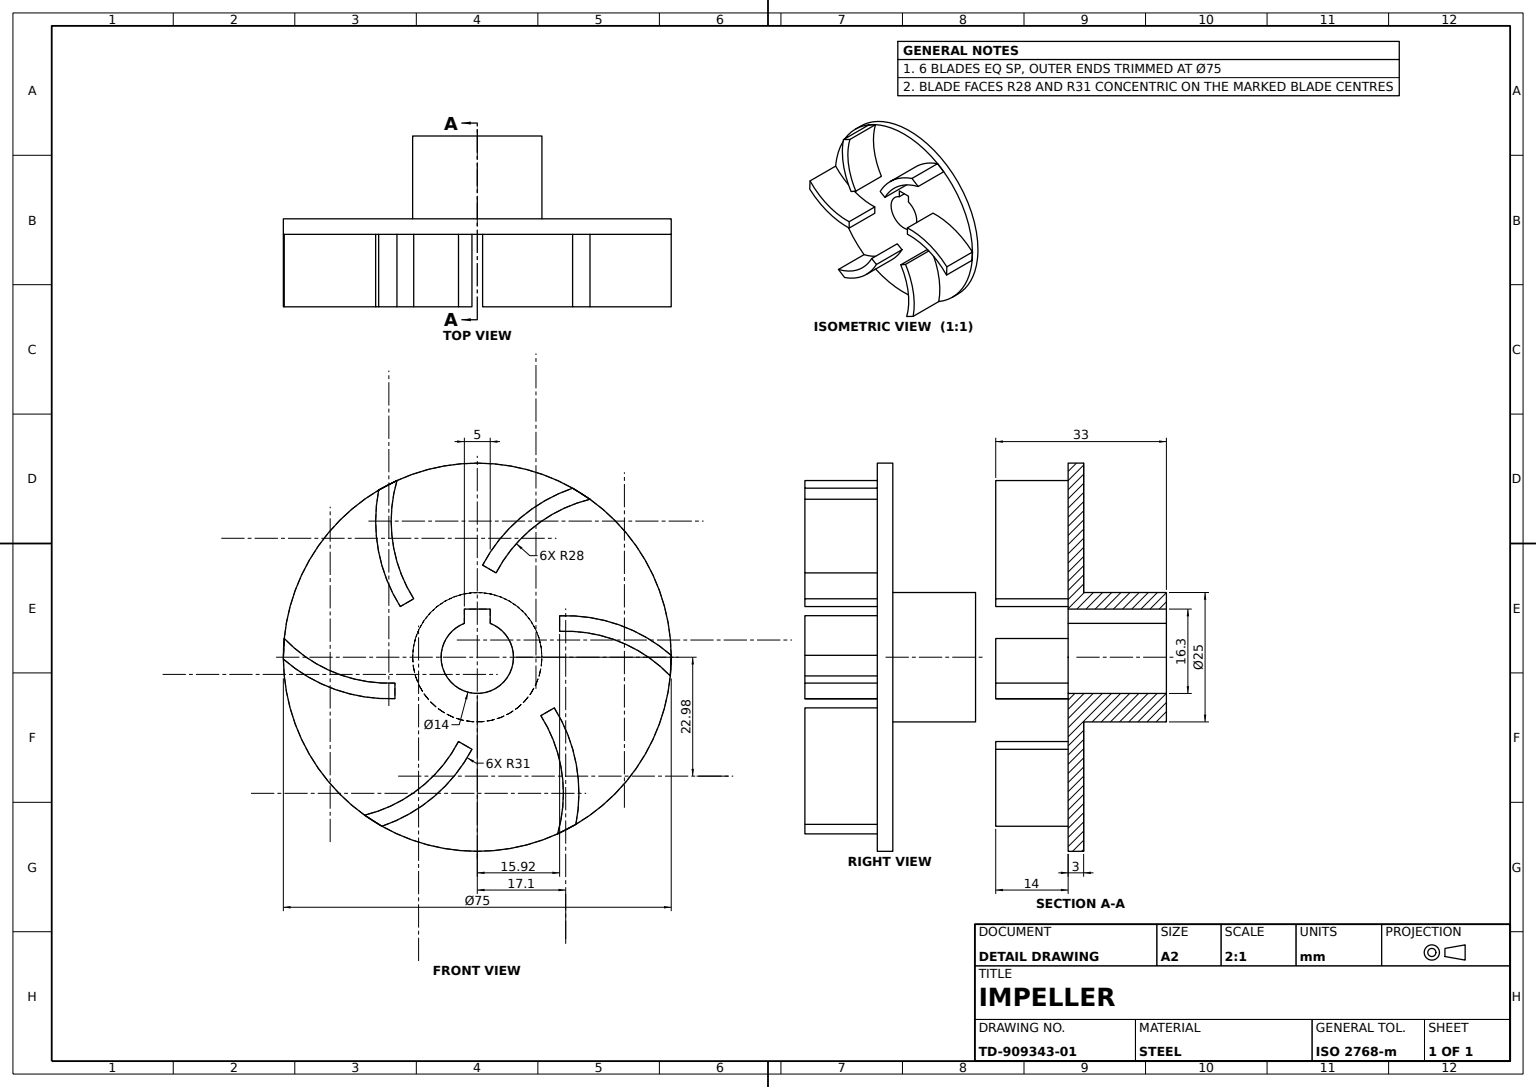
ISO-10303-21;
HEADER;
FILE_DESCRIPTION((''),'2;1');
FILE_NAME('','',(''),(''),'','','');
FILE_SCHEMA(('AUTOMOTIVE_DESIGN'));
ENDSEC;
DATA;
#1=APPLICATION_CONTEXT('');
#2=PRODUCT_CONTEXT('',#1,'mechanical');
#3=PRODUCT('','','',(#2));
#4=PRODUCT_DEFINITION_FORMATION('','',#3);
#5=PRODUCT_DEFINITION_CONTEXT('',#1,'design');
#6=PRODUCT_DEFINITION('','',#4,#5);
#7=PRODUCT_DEFINITION_SHAPE('','',#6);
#8=(LENGTH_UNIT()NAMED_UNIT(*)SI_UNIT(.MILLI.,.METRE.));
#9=(NAMED_UNIT(*)PLANE_ANGLE_UNIT()SI_UNIT($,.RADIAN.));
#10=(NAMED_UNIT(*)SI_UNIT($,.STERADIAN.)SOLID_ANGLE_UNIT());
#11=UNCERTAINTY_MEASURE_WITH_UNIT(LENGTH_MEASURE(1.E-05),#8,'distance_accuracy_value','');
#12=(GEOMETRIC_REPRESENTATION_CONTEXT(3)GLOBAL_UNCERTAINTY_ASSIGNED_CONTEXT((#11))GLOBAL_UNIT_ASSIGNED_CONTEXT((#8,#9,#10))REPRESENTATION_CONTEXT('',''));
#13=CARTESIAN_POINT('',(15.921953,5.,17.));
#14=VERTEX_POINT('',#13);
#15=CARTESIAN_POINT('',(15.921953,8.002394,17.));
#16=VERTEX_POINT('',#15);
#17=CARTESIAN_POINT('',(15.921953,0.,17.));
#18=DIRECTION('',(0.,1.,0.));
#19=VECTOR('',#18,1000.);
#20=LINE('',#17,#19);
#21=EDGE_CURVE('',#14,#16,#20,.T.);
#22=ORIENTED_EDGE('',*,*,#21,.F.);
#23=CARTESIAN_POINT('',(37.325448,-3.613988,17.));
#24=VERTEX_POINT('',#23);
#25=CARTESIAN_POINT('',(17.098232,-22.975281,17.));
#26=DIRECTION('',(0.,0.,1.));
#27=DIRECTION('',(1.,0.,0.));
#28=AXIS2_PLACEMENT_3D('',#25,#26,#27);
#29=CIRCLE('',#28,28.);
#30=EDGE_CURVE('',#24,#14,#29,.T.);
#31=ORIENTED_EDGE('',*,*,#30,.F.);
#32=CARTESIAN_POINT('',(37.498209,0.366547,17.));
#33=VERTEX_POINT('',#32);
#34=CARTESIAN_POINT('',(37.411828,-1.62372,17.));
#35=DIRECTION('',(0.043360439,0.999059494,0.));
#36=VECTOR('',#35,1000.);
#37=LINE('',#34,#36);
#38=EDGE_CURVE('',#24,#33,#37,.T.);
#39=ORIENTED_EDGE('',*,*,#38,.T.);
#40=CIRCLE('',#28,31.);
#41=EDGE_CURVE('',#33,#16,#40,.T.);
#42=ORIENTED_EDGE('',*,*,#41,.T.);
#43=EDGE_LOOP('',(#22,#31,#39,#42));
#44=FACE_OUTER_BOUND('',#43,.T.);
#45=CARTESIAN_POINT('',(0.,0.,17.));
#46=AXIS2_PLACEMENT_3D('',#45,#26,#27);
#47=PLANE('',#46);
#48=ADVANCED_FACE('',(#44),#47,.T.);
#49=CARTESIAN_POINT('',(3.630849,16.288816,17.));
#50=VERTEX_POINT('',#49);
#51=CARTESIAN_POINT('',(3.630849,16.288816,3.));
#52=VERTEX_POINT('',#51);
#53=DIRECTION('',(0.,0.,-1.));
#54=VECTOR('',#53,1000.);
#55=LINE('',#49,#54);
#56=EDGE_CURVE('',#50,#52,#55,.T.);
#57=ORIENTED_EDGE('',*,*,#56,.T.);
#58=CARTESIAN_POINT('',(21.792529,30.517793,3.));
#59=VERTEX_POINT('',#58);
#60=CARTESIAN_POINT('',(28.446293,3.319862,3.));
#61=AXIS2_PLACEMENT_3D('',#60,#26,#27);
#62=CIRCLE('',#61,28.);
#63=EDGE_CURVE('',#59,#52,#62,.T.);
#64=ORIENTED_EDGE('',*,*,#63,.F.);
#65=CARTESIAN_POINT('',(21.792529,30.517793,17.));
#66=VERTEX_POINT('',#65);
#67=LINE('',#65,#54);
#68=EDGE_CURVE('',#66,#59,#67,.T.);
#69=ORIENTED_EDGE('',*,*,#68,.F.);
#70=CARTESIAN_POINT('',(28.446293,3.319862,17.));
#71=AXIS2_PLACEMENT_3D('',#70,#26,#27);
#72=CIRCLE('',#71,28.);
#73=EDGE_CURVE('',#66,#50,#72,.T.);
#74=ORIENTED_EDGE('',*,*,#73,.T.);
#75=EDGE_LOOP('',(#57,#64,#69,#74));
#76=FACE_OUTER_BOUND('',#75,.T.);
#77=DIRECTION('',(-1.,0.,0.));
#78=AXIS2_PLACEMENT_3D('',#70,#53,#77);
#79=CYLINDRICAL_SURFACE('',#78,28.);
#80=ADVANCED_FACE('',(#76),#79,.F.);
#81=CARTESIAN_POINT('',(-3.630849,-16.288816,17.));
#82=VERTEX_POINT('',#81);
#83=CARTESIAN_POINT('',(-3.630849,-16.288816,3.));
#84=VERTEX_POINT('',#83);
#85=LINE('',#81,#54);
#86=EDGE_CURVE('',#82,#84,#85,.T.);
#87=ORIENTED_EDGE('',*,*,#86,.T.);
#88=CARTESIAN_POINT('',(-21.792529,-30.517793,3.));
#89=VERTEX_POINT('',#88);
#90=CARTESIAN_POINT('',(-28.446293,-3.319862,3.));
#91=AXIS2_PLACEMENT_3D('',#90,#26,#27);
#92=CIRCLE('',#91,28.);
#93=EDGE_CURVE('',#89,#84,#92,.T.);
#94=ORIENTED_EDGE('',*,*,#93,.F.);
#95=CARTESIAN_POINT('',(-21.792529,-30.517793,17.));
#96=VERTEX_POINT('',#95);
#97=LINE('',#95,#54);
#98=EDGE_CURVE('',#96,#89,#97,.T.);
#99=ORIENTED_EDGE('',*,*,#98,.F.);
#100=CARTESIAN_POINT('',(-28.446293,-3.319862,17.));
#101=AXIS2_PLACEMENT_3D('',#100,#26,#27);
#102=CIRCLE('',#101,28.);
#103=EDGE_CURVE('',#96,#82,#102,.T.);
#104=ORIENTED_EDGE('',*,*,#103,.T.);
#105=EDGE_LOOP('',(#87,#94,#99,#104));
#106=FACE_OUTER_BOUND('',#105,.T.);
#107=AXIS2_PLACEMENT_3D('',#100,#53,#77);
#108=CYLINDRICAL_SURFACE('',#107,28.);
#109=ADVANCED_FACE('',(#106),#108,.F.);
#110=CARTESIAN_POINT('',(37.5,0.,3.));
#111=VERTEX_POINT('',#110);
#112=CARTESIAN_POINT('',(37.498209,0.366547,3.));
#113=VERTEX_POINT('',#112);
#114=CARTESIAN_POINT('',(0.,0.,3.));
#115=AXIS2_PLACEMENT_3D('',#114,#26,#27);
#116=CIRCLE('',#115,37.5);
#117=EDGE_CURVE('',#111,#113,#116,.T.);
#118=ORIENTED_EDGE('',*,*,#117,.T.);
#119=CARTESIAN_POINT('',(37.325448,-3.613988,3.));
#120=VERTEX_POINT('',#119);
#121=CARTESIAN_POINT('',(37.411828,-1.62372,3.));
#122=LINE('',#121,#36);
#123=EDGE_CURVE('',#120,#113,#122,.T.);
#124=ORIENTED_EDGE('',*,*,#123,.F.);
#125=EDGE_CURVE('',#120,#111,#116,.T.);
#126=ORIENTED_EDGE('',*,*,#125,.T.);
#127=EDGE_LOOP('',(#118,#124,#126));
#128=FACE_OUTER_BOUND('',#127,.T.);
#129=PLANE('',#115);
#130=ADVANCED_FACE('',(#128),#129,.T.);
#131=CARTESIAN_POINT('',(-12.291103,11.288816,17.));
#132=VERTEX_POINT('',#131);
#133=CARTESIAN_POINT('',(-14.891253,9.787619,17.));
#134=VERTEX_POINT('',#133);
#135=CARTESIAN_POINT('',(-7.960976,13.788816,17.));
#136=DIRECTION('',(-0.866025404,-0.5,0.));
#137=VECTOR('',#136,1000.);
#138=LINE('',#135,#137);
#139=EDGE_CURVE('',#132,#134,#138,.T.);
#140=ORIENTED_EDGE('',*,*,#139,.F.);
#141=CARTESIAN_POINT('',(-16.651938,26.295144,17.));
#142=VERTEX_POINT('',#141);
#143=CARTESIAN_POINT('',(11.348062,26.295144,17.));
#144=AXIS2_PLACEMENT_3D('',#143,#26,#27);
#145=CIRCLE('',#144,28.);
#146=EDGE_CURVE('',#142,#132,#145,.T.);
#147=ORIENTED_EDGE('',*,*,#146,.F.);
#148=CARTESIAN_POINT('',(-15.532919,34.13178,17.));
#149=VERTEX_POINT('',#148);
#150=EDGE_CURVE('',#149,#142,#145,.T.);
#151=ORIENTED_EDGE('',*,*,#150,.F.);
#152=CARTESIAN_POINT('',(-19.066543,32.291128,17.));
#153=VERTEX_POINT('',#152);
#154=CARTESIAN_POINT('',(-17.299731,33.211454,17.));
#155=DIRECTION('',(-0.886891121,-0.461978505,0.));
#156=VECTOR('',#155,1000.);
#157=LINE('',#154,#156);
#158=EDGE_CURVE('',#149,#153,#157,.T.);
#159=ORIENTED_EDGE('',*,*,#158,.T.);
#160=CARTESIAN_POINT('',(-19.651938,26.295144,17.));
#161=VERTEX_POINT('',#160);
#162=CIRCLE('',#144,31.);
#163=EDGE_CURVE('',#153,#161,#162,.T.);
#164=ORIENTED_EDGE('',*,*,#163,.T.);
#165=EDGE_CURVE('',#161,#134,#162,.T.);
#166=ORIENTED_EDGE('',*,*,#165,.T.);
#167=EDGE_LOOP('',(#140,#147,#151,#159,#164,#166));
#168=FACE_OUTER_BOUND('',#167,.T.);
#169=ADVANCED_FACE('',(#168),#47,.T.);
#170=CARTESIAN_POINT('',(15.532919,-34.13178,17.));
#171=VERTEX_POINT('',#170);
#172=CARTESIAN_POINT('',(12.291103,-11.288816,17.));
#173=VERTEX_POINT('',#172);
#174=CARTESIAN_POINT('',(-11.348062,-26.295144,17.));
#175=AXIS2_PLACEMENT_3D('',#174,#26,#27);
#176=CIRCLE('',#175,28.);
#177=EDGE_CURVE('',#171,#173,#176,.T.);
#178=ORIENTED_EDGE('',*,*,#177,.T.);
#179=CARTESIAN_POINT('',(12.291103,-11.288816,3.));
#180=VERTEX_POINT('',#179);
#181=LINE('',#172,#54);
#182=EDGE_CURVE('',#173,#180,#181,.T.);
#183=ORIENTED_EDGE('',*,*,#182,.T.);
#184=CARTESIAN_POINT('',(15.532919,-34.13178,3.));
#185=VERTEX_POINT('',#184);
#186=CARTESIAN_POINT('',(-11.348062,-26.295144,3.));
#187=AXIS2_PLACEMENT_3D('',#186,#26,#27);
#188=CIRCLE('',#187,28.);
#189=EDGE_CURVE('',#185,#180,#188,.T.);
#190=ORIENTED_EDGE('',*,*,#189,.F.);
#191=LINE('',#170,#54);
#192=EDGE_CURVE('',#171,#185,#191,.T.);
#193=ORIENTED_EDGE('',*,*,#192,.F.);
#194=EDGE_LOOP('',(#178,#183,#190,#193));
#195=FACE_OUTER_BOUND('',#194,.T.);
#196=AXIS2_PLACEMENT_3D('',#174,#53,#77);
#197=CYLINDRICAL_SURFACE('',#196,28.);
#198=ADVANCED_FACE('',(#195),#197,.F.);
#199=CARTESIAN_POINT('',(-7.,0.,3.));
#200=VERTEX_POINT('',#199);
#201=CARTESIAN_POINT('',(-7.,0.,-16.));
#202=VERTEX_POINT('',#201);
#203=CARTESIAN_POINT('',(-7.,0.,17.));
#204=LINE('',#203,#54);
#205=EDGE_CURVE('',#200,#202,#204,.T.);
#206=ORIENTED_EDGE('',*,*,#205,.F.);
#207=CARTESIAN_POINT('',(7.,0.,3.));
#208=VERTEX_POINT('',#207);
#209=CIRCLE('',#115,7.);
#210=EDGE_CURVE('',#200,#208,#209,.T.);
#211=ORIENTED_EDGE('',*,*,#210,.T.);
#212=CARTESIAN_POINT('',(7.,0.,-16.));
#213=VERTEX_POINT('',#212);
#214=CARTESIAN_POINT('',(7.,0.,17.));
#215=LINE('',#214,#54);
#216=EDGE_CURVE('',#208,#213,#215,.T.);
#217=ORIENTED_EDGE('',*,*,#216,.T.);
#218=CARTESIAN_POINT('',(0.,0.,-16.));
#219=AXIS2_PLACEMENT_3D('',#218,#53,#77);
#220=CIRCLE('',#219,7.);
#221=EDGE_CURVE('',#213,#202,#220,.T.);
#222=ORIENTED_EDGE('',*,*,#221,.T.);
#223=EDGE_LOOP('',(#206,#211,#217,#222));
#224=FACE_OUTER_BOUND('',#223,.T.);
#225=AXIS2_PLACEMENT_3D('',#45,#53,#77);
#226=CYLINDRICAL_SURFACE('',#225,7.);
#227=ADVANCED_FACE('',(#224),#226,.F.);
#228=CARTESIAN_POINT('',(1.0307,17.790013,3.));
#229=VERTEX_POINT('',#228);
#230=CARTESIAN_POINT('',(7.960976,13.788816,3.));
#231=DIRECTION('',(-0.866025404,0.5,0.));
#232=VECTOR('',#231,1000.);
#233=LINE('',#230,#232);
#234=EDGE_CURVE('',#52,#229,#233,.T.);
#235=ORIENTED_EDGE('',*,*,#234,.F.);
#236=ORIENTED_EDGE('',*,*,#56,.F.);
#237=CARTESIAN_POINT('',(1.0307,17.790013,17.));
#238=VERTEX_POINT('',#237);
#239=CARTESIAN_POINT('',(7.960976,13.788816,17.));
#240=LINE('',#239,#232);
#241=EDGE_CURVE('',#50,#238,#240,.T.);
#242=ORIENTED_EDGE('',*,*,#241,.T.);
#243=LINE('',#237,#54);
#244=EDGE_CURVE('',#238,#229,#243,.T.);
#245=ORIENTED_EDGE('',*,*,#244,.T.);
#246=EDGE_LOOP('',(#235,#236,#242,#245));
#247=FACE_OUTER_BOUND('',#246,.T.);
#248=DIRECTION('',(-0.5,-0.866025404,0.));
#249=DIRECTION('',(0.866025404,-0.5,0.));
#250=AXIS2_PLACEMENT_3D('',#239,#248,#249);
#251=PLANE('',#250);
#252=ADVANCED_FACE('',(#247),#251,.T.);
#253=CARTESIAN_POINT('',(-2.5,6.538348,3.));
#254=VERTEX_POINT('',#253);
#255=EDGE_CURVE('',#254,#200,#209,.T.);
#256=ORIENTED_EDGE('',*,*,#255,.T.);
#257=ORIENTED_EDGE('',*,*,#205,.T.);
#258=CARTESIAN_POINT('',(-2.5,6.538348,-16.));
#259=VERTEX_POINT('',#258);
#260=EDGE_CURVE('',#202,#259,#220,.T.);
#261=ORIENTED_EDGE('',*,*,#260,.T.);
#262=CARTESIAN_POINT('',(-2.5,6.538348,17.));
#263=LINE('',#262,#54);
#264=EDGE_CURVE('',#254,#259,#263,.T.);
#265=ORIENTED_EDGE('',*,*,#264,.F.);
#266=EDGE_LOOP('',(#256,#257,#261,#265));
#267=FACE_OUTER_BOUND('',#266,.T.);
#268=ADVANCED_FACE('',(#267),#226,.F.);
#269=CARTESIAN_POINT('',(-18.431666,-32.657675,17.));
#270=VERTEX_POINT('',#269);
#271=CARTESIAN_POINT('',(-18.431666,-32.657675,3.));
#272=VERTEX_POINT('',#271);
#273=LINE('',#269,#54);
#274=EDGE_CURVE('',#270,#272,#273,.T.);
#275=ORIENTED_EDGE('',*,*,#274,.T.);
#276=CARTESIAN_POINT('',(-1.0307,-17.790013,3.));
#277=VERTEX_POINT('',#276);
#278=CIRCLE('',#91,31.);
#279=EDGE_CURVE('',#272,#277,#278,.T.);
#280=ORIENTED_EDGE('',*,*,#279,.T.);
#281=CARTESIAN_POINT('',(-1.0307,-17.790013,17.));
#282=VERTEX_POINT('',#281);
#283=LINE('',#281,#54);
#284=EDGE_CURVE('',#282,#277,#283,.T.);
#285=ORIENTED_EDGE('',*,*,#284,.F.);
#286=CIRCLE('',#101,31.);
#287=EDGE_CURVE('',#270,#282,#286,.T.);
#288=ORIENTED_EDGE('',*,*,#287,.F.);
#289=EDGE_LOOP('',(#275,#280,#285,#288));
#290=FACE_OUTER_BOUND('',#289,.T.);
#291=CYLINDRICAL_SURFACE('',#107,31.);
#292=ADVANCED_FACE('',(#290),#291,.T.);
#293=CARTESIAN_POINT('',(-19.651938,26.295144,3.));
#294=VERTEX_POINT('',#293);
#295=LINE('',#160,#54);
#296=EDGE_CURVE('',#161,#294,#295,.T.);
#297=ORIENTED_EDGE('',*,*,#296,.T.);
#298=CARTESIAN_POINT('',(-14.891253,9.787619,3.));
#299=VERTEX_POINT('',#298);
#300=CARTESIAN_POINT('',(11.348062,26.295144,3.));
#301=AXIS2_PLACEMENT_3D('',#300,#26,#27);
#302=CIRCLE('',#301,31.);
#303=EDGE_CURVE('',#294,#299,#302,.T.);
#304=ORIENTED_EDGE('',*,*,#303,.T.);
#305=LINE('',#133,#54);
#306=EDGE_CURVE('',#134,#299,#305,.T.);
#307=ORIENTED_EDGE('',*,*,#306,.F.);
#308=ORIENTED_EDGE('',*,*,#165,.F.);
#309=EDGE_LOOP('',(#297,#304,#307,#308));
#310=FACE_OUTER_BOUND('',#309,.T.);
#311=AXIS2_PLACEMENT_3D('',#143,#53,#77);
#312=CYLINDRICAL_SURFACE('',#311,31.);
#313=ADVANCED_FACE('',(#310),#312,.T.);
#314=CARTESIAN_POINT('',(14.891253,-9.787619,17.));
#315=VERTEX_POINT('',#314);
#316=CARTESIAN_POINT('',(14.891253,-9.787619,3.));
#317=VERTEX_POINT('',#316);
#318=LINE('',#314,#54);
#319=EDGE_CURVE('',#315,#317,#318,.T.);
#320=ORIENTED_EDGE('',*,*,#319,.F.);
#321=CARTESIAN_POINT('',(19.066543,-32.291128,17.));
#322=VERTEX_POINT('',#321);
#323=CIRCLE('',#175,31.);
#324=EDGE_CURVE('',#322,#315,#323,.T.);
#325=ORIENTED_EDGE('',*,*,#324,.F.);
#326=CARTESIAN_POINT('',(19.066543,-32.291128,3.));
#327=VERTEX_POINT('',#326);
#328=LINE('',#321,#54);
#329=EDGE_CURVE('',#322,#327,#328,.T.);
#330=ORIENTED_EDGE('',*,*,#329,.T.);
#331=CIRCLE('',#187,31.);
#332=EDGE_CURVE('',#327,#317,#331,.T.);
#333=ORIENTED_EDGE('',*,*,#332,.T.);
#334=EDGE_LOOP('',(#320,#325,#330,#333));
#335=FACE_OUTER_BOUND('',#334,.T.);
#336=CYLINDRICAL_SURFACE('',#196,31.);
#337=ADVANCED_FACE('',(#335),#336,.T.);
#338=CARTESIAN_POINT('',(2.5,9.3,3.));
#339=VERTEX_POINT('',#338);
#340=CARTESIAN_POINT('',(-2.5,9.3,3.));
#341=VERTEX_POINT('',#340);
#342=CARTESIAN_POINT('',(0.,9.3,3.));
#343=VECTOR('',#77,1000.);
#344=LINE('',#342,#343);
#345=EDGE_CURVE('',#339,#341,#344,.T.);
#346=ORIENTED_EDGE('',*,*,#345,.T.);
#347=CARTESIAN_POINT('',(-2.5,9.3,-16.));
#348=VERTEX_POINT('',#347);
#349=CARTESIAN_POINT('',(-2.5,9.3,17.));
#350=LINE('',#349,#54);
#351=EDGE_CURVE('',#341,#348,#350,.T.);
#352=ORIENTED_EDGE('',*,*,#351,.T.);
#353=CARTESIAN_POINT('',(2.5,9.3,-16.));
#354=VERTEX_POINT('',#353);
#355=VECTOR('',#27,1000.);
#356=LINE('',#353,#355);
#357=EDGE_CURVE('',#348,#354,#356,.T.);
#358=ORIENTED_EDGE('',*,*,#357,.T.);
#359=CARTESIAN_POINT('',(2.5,9.3,17.));
#360=LINE('',#359,#54);
#361=EDGE_CURVE('',#339,#354,#360,.T.);
#362=ORIENTED_EDGE('',*,*,#361,.F.);
#363=EDGE_LOOP('',(#346,#352,#358,#362));
#364=FACE_OUTER_BOUND('',#363,.T.);
#365=AXIS2_PLACEMENT_3D('',#359,#18,#26);
#366=PLANE('',#365);
#367=ADVANCED_FACE('',(#364),#366,.F.);
#368=CARTESIAN_POINT('',(37.5,0.,0.));
#369=VERTEX_POINT('',#368);
#370=LINE('',#110,#54);
#371=EDGE_CURVE('',#111,#369,#370,.T.);
#372=ORIENTED_EDGE('',*,*,#371,.T.);
#373=CARTESIAN_POINT('',(-37.5,0.,0.));
#374=VERTEX_POINT('',#373);
#375=CARTESIAN_POINT('',(0.,0.,0.));
#376=AXIS2_PLACEMENT_3D('',#375,#26,#27);
#377=CIRCLE('',#376,37.5);
#378=EDGE_CURVE('',#369,#374,#377,.T.);
#379=ORIENTED_EDGE('',*,*,#378,.T.);
#380=CARTESIAN_POINT('',(-37.5,0.,3.));
#381=VERTEX_POINT('',#380);
#382=LINE('',#380,#54);
#383=EDGE_CURVE('',#381,#374,#382,.T.);
#384=ORIENTED_EDGE('',*,*,#383,.F.);
#385=CARTESIAN_POINT('',(-37.325448,3.613988,3.));
#386=VERTEX_POINT('',#385);
#387=EDGE_CURVE('',#386,#381,#116,.T.);
#388=ORIENTED_EDGE('',*,*,#387,.F.);
#389=CARTESIAN_POINT('',(-19.066543,32.291128,3.));
#390=VERTEX_POINT('',#389);
#391=EDGE_CURVE('',#390,#386,#116,.T.);
#392=ORIENTED_EDGE('',*,*,#391,.F.);
#393=CARTESIAN_POINT('',(-15.532919,34.13178,3.));
#394=VERTEX_POINT('',#393);
#395=EDGE_CURVE('',#394,#390,#116,.T.);
#396=ORIENTED_EDGE('',*,*,#395,.F.);
#397=CARTESIAN_POINT('',(18.431666,32.657675,3.));
#398=VERTEX_POINT('',#397);
#399=EDGE_CURVE('',#398,#394,#116,.T.);
#400=ORIENTED_EDGE('',*,*,#399,.F.);
#401=EDGE_CURVE('',#59,#398,#116,.T.);
#402=ORIENTED_EDGE('',*,*,#401,.F.);
#403=EDGE_CURVE('',#113,#59,#116,.T.);
#404=ORIENTED_EDGE('',*,*,#403,.F.);
#405=ORIENTED_EDGE('',*,*,#117,.F.);
#406=EDGE_LOOP('',(#372,#379,#384,#388,#392,#396,#400,#402,#404,#405));
#407=FACE_OUTER_BOUND('',#406,.T.);
#408=AXIS2_PLACEMENT_3D('',#114,#53,#77);
#409=CYLINDRICAL_SURFACE('',#408,37.5);
#410=ADVANCED_FACE('',(#407),#409,.T.);
#411=CARTESIAN_POINT('',(2.5,6.538348,3.));
#412=VERTEX_POINT('',#411);
#413=EDGE_CURVE('',#208,#412,#209,.T.);
#414=ORIENTED_EDGE('',*,*,#413,.T.);
#415=CARTESIAN_POINT('',(2.5,6.538348,-16.));
#416=VERTEX_POINT('',#415);
#417=CARTESIAN_POINT('',(2.5,6.538348,17.));
#418=LINE('',#417,#54);
#419=EDGE_CURVE('',#412,#416,#418,.T.);
#420=ORIENTED_EDGE('',*,*,#419,.T.);
#421=EDGE_CURVE('',#416,#213,#220,.T.);
#422=ORIENTED_EDGE('',*,*,#421,.T.);
#423=ORIENTED_EDGE('',*,*,#216,.F.);
#424=EDGE_LOOP('',(#414,#420,#422,#423));
#425=FACE_OUTER_BOUND('',#424,.T.);
#426=ADVANCED_FACE('',(#425),#226,.F.);
#427=CARTESIAN_POINT('',(-7.960976,-13.788816,3.));
#428=VECTOR('',#249,1000.);
#429=LINE('',#427,#428);
#430=EDGE_CURVE('',#84,#277,#429,.T.);
#431=ORIENTED_EDGE('',*,*,#430,.F.);
#432=ORIENTED_EDGE('',*,*,#86,.F.);
#433=CARTESIAN_POINT('',(-7.960976,-13.788816,17.));
#434=LINE('',#433,#428);
#435=EDGE_CURVE('',#82,#282,#434,.T.);
#436=ORIENTED_EDGE('',*,*,#435,.T.);
#437=ORIENTED_EDGE('',*,*,#284,.T.);
#438=EDGE_LOOP('',(#431,#432,#436,#437));
#439=FACE_OUTER_BOUND('',#438,.T.);
#440=DIRECTION('',(0.5,0.866025404,0.));
#441=AXIS2_PLACEMENT_3D('',#433,#440,#231);
#442=PLANE('',#441);
#443=ADVANCED_FACE('',(#439),#442,.T.);
#444=CARTESIAN_POINT('',(18.431666,32.657675,17.));
#445=VERTEX_POINT('',#444);
#446=CIRCLE('',#71,31.);
#447=EDGE_CURVE('',#445,#238,#446,.T.);
#448=ORIENTED_EDGE('',*,*,#447,.F.);
#449=LINE('',#444,#54);
#450=EDGE_CURVE('',#445,#398,#449,.T.);
#451=ORIENTED_EDGE('',*,*,#450,.T.);
#452=CIRCLE('',#61,31.);
#453=EDGE_CURVE('',#398,#229,#452,.T.);
#454=ORIENTED_EDGE('',*,*,#453,.T.);
#455=ORIENTED_EDGE('',*,*,#244,.F.);
#456=EDGE_LOOP('',(#448,#451,#454,#455));
#457=FACE_OUTER_BOUND('',#456,.T.);
#458=CYLINDRICAL_SURFACE('',#78,31.);
#459=ADVANCED_FACE('',(#457),#458,.T.);
#460=ORIENTED_EDGE('',*,*,#163,.F.);
#461=LINE('',#152,#54);
#462=EDGE_CURVE('',#153,#390,#461,.T.);
#463=ORIENTED_EDGE('',*,*,#462,.T.);
#464=EDGE_CURVE('',#390,#294,#302,.T.);
#465=ORIENTED_EDGE('',*,*,#464,.T.);
#466=ORIENTED_EDGE('',*,*,#296,.F.);
#467=EDGE_LOOP('',(#460,#463,#465,#466));
#468=FACE_OUTER_BOUND('',#467,.T.);
#469=ADVANCED_FACE('',(#468),#312,.T.);
#470=ORIENTED_EDGE('',*,*,#306,.T.);
#471=CARTESIAN_POINT('',(-12.291103,11.288816,3.));
#472=VERTEX_POINT('',#471);
#473=CARTESIAN_POINT('',(-7.960976,13.788816,3.));
#474=LINE('',#473,#137);
#475=EDGE_CURVE('',#472,#299,#474,.T.);
#476=ORIENTED_EDGE('',*,*,#475,.F.);
#477=LINE('',#131,#54);
#478=EDGE_CURVE('',#132,#472,#477,.T.);
#479=ORIENTED_EDGE('',*,*,#478,.F.);
#480=ORIENTED_EDGE('',*,*,#139,.T.);
#481=EDGE_LOOP('',(#470,#476,#479,#480));
#482=FACE_OUTER_BOUND('',#481,.T.);
#483=DIRECTION('',(0.5,-0.866025404,0.));
#484=DIRECTION('',(0.866025404,0.5,0.));
#485=AXIS2_PLACEMENT_3D('',#135,#483,#484);
#486=PLANE('',#485);
#487=ADVANCED_FACE('',(#482),#486,.T.);
#488=CARTESIAN_POINT('',(-20.112097,-31.587734,17.));
#489=DIRECTION('',(0.843530682,-0.537080988,0.));
#490=VECTOR('',#489,1000.);
#491=LINE('',#488,#490);
#492=EDGE_CURVE('',#96,#270,#491,.T.);
#493=ORIENTED_EDGE('',*,*,#492,.F.);
#494=ORIENTED_EDGE('',*,*,#98,.T.);
#495=CARTESIAN_POINT('',(-20.112097,-31.587734,3.));
#496=LINE('',#495,#490);
#497=EDGE_CURVE('',#89,#272,#496,.T.);
#498=ORIENTED_EDGE('',*,*,#497,.T.);
#499=ORIENTED_EDGE('',*,*,#274,.F.);
#500=EDGE_LOOP('',(#493,#494,#498,#499));
#501=FACE_OUTER_BOUND('',#500,.T.);
#502=DIRECTION('',(0.537080988,0.843530682,0.));
#503=DIRECTION('',(-0.843530682,0.537080988,0.));
#504=AXIS2_PLACEMENT_3D('',#488,#502,#503);
#505=PLANE('',#504);
#506=ADVANCED_FACE('',(#501),#505,.F.);
#507=ORIENTED_EDGE('',*,*,#395,.T.);
#508=CARTESIAN_POINT('',(-17.299731,33.211454,3.));
#509=LINE('',#508,#156);
#510=EDGE_CURVE('',#394,#390,#509,.T.);
#511=ORIENTED_EDGE('',*,*,#510,.F.);
#512=EDGE_LOOP('',(#507,#511));
#513=FACE_OUTER_BOUND('',#512,.T.);
#514=ADVANCED_FACE('',(#513),#129,.T.);
#515=ORIENTED_EDGE('',*,*,#68,.T.);
#516=CARTESIAN_POINT('',(20.112097,31.587734,3.));
#517=VECTOR('',#503,1000.);
#518=LINE('',#516,#517);
#519=EDGE_CURVE('',#59,#398,#518,.T.);
#520=ORIENTED_EDGE('',*,*,#519,.T.);
#521=ORIENTED_EDGE('',*,*,#450,.F.);
#522=CARTESIAN_POINT('',(20.112097,31.587734,17.));
#523=LINE('',#522,#517);
#524=EDGE_CURVE('',#66,#445,#523,.T.);
#525=ORIENTED_EDGE('',*,*,#524,.F.);
#526=EDGE_LOOP('',(#515,#520,#521,#525));
#527=FACE_OUTER_BOUND('',#526,.T.);
#528=DIRECTION('',(-0.537080988,-0.843530682,0.));
#529=AXIS2_PLACEMENT_3D('',#522,#528,#489);
#530=PLANE('',#529);
#531=ADVANCED_FACE('',(#527),#530,.F.);
#532=ORIENTED_EDGE('',*,*,#324,.T.);
#533=CARTESIAN_POINT('',(7.960976,-13.788816,17.));
#534=VECTOR('',#484,1000.);
#535=LINE('',#533,#534);
#536=EDGE_CURVE('',#173,#315,#535,.T.);
#537=ORIENTED_EDGE('',*,*,#536,.F.);
#538=ORIENTED_EDGE('',*,*,#177,.F.);
#539=CARTESIAN_POINT('',(17.299731,-33.211454,17.));
#540=DIRECTION('',(0.886891121,0.461978505,0.));
#541=VECTOR('',#540,1000.);
#542=LINE('',#539,#541);
#543=EDGE_CURVE('',#171,#322,#542,.T.);
#544=ORIENTED_EDGE('',*,*,#543,.T.);
#545=EDGE_LOOP('',(#532,#537,#538,#544));
#546=FACE_OUTER_BOUND('',#545,.T.);
#547=ADVANCED_FACE('',(#546),#47,.T.);
#548=CARTESIAN_POINT('',(-37.498209,-0.366547,17.));
#549=VERTEX_POINT('',#548);
#550=CARTESIAN_POINT('',(-15.921953,-8.002394,17.));
#551=VERTEX_POINT('',#550);
#552=CARTESIAN_POINT('',(-17.098232,22.975281,17.));
#553=AXIS2_PLACEMENT_3D('',#552,#26,#27);
#554=CIRCLE('',#553,31.);
#555=EDGE_CURVE('',#549,#551,#554,.T.);
#556=ORIENTED_EDGE('',*,*,#555,.T.);
#557=CARTESIAN_POINT('',(-15.921953,-5.,17.));
#558=VERTEX_POINT('',#557);
#559=CARTESIAN_POINT('',(-15.921953,0.,17.));
#560=DIRECTION('',(0.,-1.,0.));
#561=VECTOR('',#560,1000.);
#562=LINE('',#559,#561);
#563=EDGE_CURVE('',#558,#551,#562,.T.);
#564=ORIENTED_EDGE('',*,*,#563,.F.);
#565=CARTESIAN_POINT('',(-37.325448,3.613988,17.));
#566=VERTEX_POINT('',#565);
#567=CIRCLE('',#553,28.);
#568=EDGE_CURVE('',#566,#558,#567,.T.);
#569=ORIENTED_EDGE('',*,*,#568,.F.);
#570=CARTESIAN_POINT('',(-37.411828,1.62372,17.));
#571=DIRECTION('',(-0.043360439,-0.999059494,0.));
#572=VECTOR('',#571,1000.);
#573=LINE('',#570,#572);
#574=EDGE_CURVE('',#566,#549,#573,.T.);
#575=ORIENTED_EDGE('',*,*,#574,.T.);
#576=EDGE_LOOP('',(#556,#564,#569,#575));
#577=FACE_OUTER_BOUND('',#576,.T.);
#578=ADVANCED_FACE('',(#577),#47,.T.);
#579=ORIENTED_EDGE('',*,*,#413,.F.);
#580=ORIENTED_EDGE('',*,*,#210,.F.);
#581=ORIENTED_EDGE('',*,*,#255,.F.);
#582=CARTESIAN_POINT('',(-2.5,0.,3.));
#583=LINE('',#582,#561);
#584=EDGE_CURVE('',#341,#254,#583,.T.);
#585=ORIENTED_EDGE('',*,*,#584,.F.);
#586=ORIENTED_EDGE('',*,*,#345,.F.);
#587=CARTESIAN_POINT('',(2.5,0.,3.));
#588=LINE('',#587,#19);
#589=EDGE_CURVE('',#412,#339,#588,.T.);
#590=ORIENTED_EDGE('',*,*,#589,.F.);
#591=EDGE_LOOP('',(#579,#580,#581,#585,#586,#590));
#592=FACE_BOUND('',#591,.T.);
#593=CARTESIAN_POINT('',(-37.498209,-0.366547,3.));
#594=VERTEX_POINT('',#593);
#595=CARTESIAN_POINT('',(-15.921953,-8.002394,3.));
#596=VERTEX_POINT('',#595);
#597=CARTESIAN_POINT('',(-17.098232,22.975281,3.));
#598=AXIS2_PLACEMENT_3D('',#597,#26,#27);
#599=CIRCLE('',#598,31.);
#600=EDGE_CURVE('',#594,#596,#599,.T.);
#601=ORIENTED_EDGE('',*,*,#600,.F.);
#602=EDGE_CURVE('',#594,#89,#116,.T.);
#603=ORIENTED_EDGE('',*,*,#602,.T.);
#604=ORIENTED_EDGE('',*,*,#93,.T.);
#605=ORIENTED_EDGE('',*,*,#430,.T.);
#606=ORIENTED_EDGE('',*,*,#279,.F.);
#607=EDGE_CURVE('',#272,#185,#116,.T.);
#608=ORIENTED_EDGE('',*,*,#607,.T.);
#609=ORIENTED_EDGE('',*,*,#189,.T.);
#610=CARTESIAN_POINT('',(7.960976,-13.788816,3.));
#611=LINE('',#610,#534);
#612=EDGE_CURVE('',#180,#317,#611,.T.);
#613=ORIENTED_EDGE('',*,*,#612,.T.);
#614=ORIENTED_EDGE('',*,*,#332,.F.);
#615=EDGE_CURVE('',#327,#120,#116,.T.);
#616=ORIENTED_EDGE('',*,*,#615,.T.);
#617=CARTESIAN_POINT('',(15.921953,5.,3.));
#618=VERTEX_POINT('',#617);
#619=CARTESIAN_POINT('',(17.098232,-22.975281,3.));
#620=AXIS2_PLACEMENT_3D('',#619,#26,#27);
#621=CIRCLE('',#620,28.);
#622=EDGE_CURVE('',#120,#618,#621,.T.);
#623=ORIENTED_EDGE('',*,*,#622,.T.);
#624=CARTESIAN_POINT('',(15.921953,8.002394,3.));
#625=VERTEX_POINT('',#624);
#626=CARTESIAN_POINT('',(15.921953,0.,3.));
#627=LINE('',#626,#19);
#628=EDGE_CURVE('',#618,#625,#627,.T.);
#629=ORIENTED_EDGE('',*,*,#628,.T.);
#630=CIRCLE('',#620,31.);
#631=EDGE_CURVE('',#113,#625,#630,.T.);
#632=ORIENTED_EDGE('',*,*,#631,.F.);
#633=ORIENTED_EDGE('',*,*,#403,.T.);
#634=ORIENTED_EDGE('',*,*,#63,.T.);
#635=ORIENTED_EDGE('',*,*,#234,.T.);
#636=ORIENTED_EDGE('',*,*,#453,.F.);
#637=ORIENTED_EDGE('',*,*,#399,.T.);
#638=CARTESIAN_POINT('',(-16.651938,26.295144,3.));
#639=VERTEX_POINT('',#638);
#640=CIRCLE('',#301,28.);
#641=EDGE_CURVE('',#394,#639,#640,.T.);
#642=ORIENTED_EDGE('',*,*,#641,.T.);
#643=EDGE_CURVE('',#639,#472,#640,.T.);
#644=ORIENTED_EDGE('',*,*,#643,.T.);
#645=ORIENTED_EDGE('',*,*,#475,.T.);
#646=ORIENTED_EDGE('',*,*,#303,.F.);
#647=ORIENTED_EDGE('',*,*,#464,.F.);
#648=ORIENTED_EDGE('',*,*,#391,.T.);
#649=CARTESIAN_POINT('',(-15.921953,-5.,3.));
#650=VERTEX_POINT('',#649);
#651=CIRCLE('',#598,28.);
#652=EDGE_CURVE('',#386,#650,#651,.T.);
#653=ORIENTED_EDGE('',*,*,#652,.T.);
#654=CARTESIAN_POINT('',(-15.921953,0.,3.));
#655=LINE('',#654,#561);
#656=EDGE_CURVE('',#650,#596,#655,.T.);
#657=ORIENTED_EDGE('',*,*,#656,.T.);
#658=EDGE_LOOP('',(#601,#603,#604,#605,#606,#608,#609,#613,#614,#616,#623,#629,#632,#633,#634,#635,#636,#637,#642,#644,#645,#646,#647,#648,#653,#657));
#659=FACE_OUTER_BOUND('',#658,.T.);
#660=ADVANCED_FACE('',(#592,#659),#129,.T.);
#661=CARTESIAN_POINT('',(12.5,0.,-16.));
#662=VERTEX_POINT('',#661);
#663=CARTESIAN_POINT('',(-12.5,0.,-16.));
#664=VERTEX_POINT('',#663);
#665=CIRCLE('',#219,12.5);
#666=EDGE_CURVE('',#662,#664,#665,.T.);
#667=ORIENTED_EDGE('',*,*,#666,.F.);
#668=CARTESIAN_POINT('',(12.5,0.,0.));
#669=VERTEX_POINT('',#668);
#670=VECTOR('',#26,1000.);
#671=LINE('',#661,#670);
#672=EDGE_CURVE('',#662,#669,#671,.T.);
#673=ORIENTED_EDGE('',*,*,#672,.T.);
#674=CARTESIAN_POINT('',(-12.5,0.,0.));
#675=VERTEX_POINT('',#674);
#676=AXIS2_PLACEMENT_3D('',#375,#53,#77);
#677=CIRCLE('',#676,12.5);
#678=EDGE_CURVE('',#669,#675,#677,.T.);
#679=ORIENTED_EDGE('',*,*,#678,.T.);
#680=LINE('',#663,#670);
#681=EDGE_CURVE('',#664,#675,#680,.T.);
#682=ORIENTED_EDGE('',*,*,#681,.F.);
#683=EDGE_LOOP('',(#667,#673,#679,#682));
#684=FACE_OUTER_BOUND('',#683,.T.);
#685=AXIS2_PLACEMENT_3D('',#218,#26,#27);
#686=CYLINDRICAL_SURFACE('',#685,12.5);
#687=ADVANCED_FACE('',(#684),#686,.T.);
#688=ORIENTED_EDGE('',*,*,#401,.T.);
#689=ORIENTED_EDGE('',*,*,#519,.F.);
#690=EDGE_LOOP('',(#688,#689));
#691=FACE_OUTER_BOUND('',#690,.T.);
#692=ADVANCED_FACE('',(#691),#129,.T.);
#693=ORIENTED_EDGE('',*,*,#563,.T.);
#694=LINE('',#550,#54);
#695=EDGE_CURVE('',#551,#596,#694,.T.);
#696=ORIENTED_EDGE('',*,*,#695,.T.);
#697=ORIENTED_EDGE('',*,*,#656,.F.);
#698=LINE('',#557,#54);
#699=EDGE_CURVE('',#558,#650,#698,.T.);
#700=ORIENTED_EDGE('',*,*,#699,.F.);
#701=EDGE_LOOP('',(#693,#696,#697,#700));
#702=FACE_OUTER_BOUND('',#701,.T.);
#703=AXIS2_PLACEMENT_3D('',#559,#27,#53);
#704=PLANE('',#703);
#705=ADVANCED_FACE('',(#702),#704,.T.);
#706=EDGE_CURVE('',#185,#327,#116,.T.);
#707=ORIENTED_EDGE('',*,*,#706,.T.);
#708=CARTESIAN_POINT('',(17.299731,-33.211454,3.));
#709=LINE('',#708,#541);
#710=EDGE_CURVE('',#185,#327,#709,.T.);
#711=ORIENTED_EDGE('',*,*,#710,.F.);
#712=EDGE_LOOP('',(#707,#711));
#713=FACE_OUTER_BOUND('',#712,.T.);
#714=ADVANCED_FACE('',(#713),#129,.T.);
#715=EDGE_CURVE('',#664,#662,#665,.T.);
#716=ORIENTED_EDGE('',*,*,#715,.F.);
#717=ORIENTED_EDGE('',*,*,#681,.T.);
#718=EDGE_CURVE('',#675,#669,#677,.T.);
#719=ORIENTED_EDGE('',*,*,#718,.T.);
#720=ORIENTED_EDGE('',*,*,#672,.F.);
#721=EDGE_LOOP('',(#716,#717,#719,#720));
#722=FACE_OUTER_BOUND('',#721,.T.);
#723=ADVANCED_FACE('',(#722),#686,.T.);
#724=ORIENTED_EDGE('',*,*,#447,.T.);
#725=ORIENTED_EDGE('',*,*,#241,.F.);
#726=ORIENTED_EDGE('',*,*,#73,.F.);
#727=ORIENTED_EDGE('',*,*,#524,.T.);
#728=EDGE_LOOP('',(#724,#725,#726,#727));
#729=FACE_OUTER_BOUND('',#728,.T.);
#730=ADVANCED_FACE('',(#729),#47,.T.);
#731=ORIENTED_EDGE('',*,*,#146,.T.);
#732=ORIENTED_EDGE('',*,*,#478,.T.);
#733=ORIENTED_EDGE('',*,*,#643,.F.);
#734=LINE('',#141,#54);
#735=EDGE_CURVE('',#142,#639,#734,.T.);
#736=ORIENTED_EDGE('',*,*,#735,.F.);
#737=EDGE_LOOP('',(#731,#732,#733,#736));
#738=FACE_OUTER_BOUND('',#737,.T.);
#739=CYLINDRICAL_SURFACE('',#311,28.);
#740=ADVANCED_FACE('',(#738),#739,.F.);
#741=ORIENTED_EDGE('',*,*,#510,.T.);
#742=ORIENTED_EDGE('',*,*,#462,.F.);
#743=ORIENTED_EDGE('',*,*,#158,.F.);
#744=LINE('',#148,#54);
#745=EDGE_CURVE('',#149,#394,#744,.T.);
#746=ORIENTED_EDGE('',*,*,#745,.T.);
#747=EDGE_LOOP('',(#741,#742,#743,#746));
#748=FACE_OUTER_BOUND('',#747,.T.);
#749=DIRECTION('',(0.461978505,-0.886891121,0.));
#750=AXIS2_PLACEMENT_3D('',#154,#749,#540);
#751=PLANE('',#750);
#752=ADVANCED_FACE('',(#748),#751,.F.);
#753=ORIENTED_EDGE('',*,*,#123,.T.);
#754=LINE('',#32,#54);
#755=EDGE_CURVE('',#33,#113,#754,.T.);
#756=ORIENTED_EDGE('',*,*,#755,.F.);
#757=ORIENTED_EDGE('',*,*,#38,.F.);
#758=LINE('',#23,#54);
#759=EDGE_CURVE('',#24,#120,#758,.T.);
#760=ORIENTED_EDGE('',*,*,#759,.T.);
#761=EDGE_LOOP('',(#753,#756,#757,#760));
#762=FACE_OUTER_BOUND('',#761,.T.);
#763=DIRECTION('',(-0.999059494,0.043360439,0.));
#764=AXIS2_PLACEMENT_3D('',#34,#763,#571);
#765=PLANE('',#764);
#766=ADVANCED_FACE('',(#762),#765,.F.);
#767=ORIENTED_EDGE('',*,*,#652,.F.);
#768=LINE('',#565,#54);
#769=EDGE_CURVE('',#566,#386,#768,.T.);
#770=ORIENTED_EDGE('',*,*,#769,.F.);
#771=ORIENTED_EDGE('',*,*,#568,.T.);
#772=ORIENTED_EDGE('',*,*,#699,.T.);
#773=EDGE_LOOP('',(#767,#770,#771,#772));
#774=FACE_OUTER_BOUND('',#773,.T.);
#775=AXIS2_PLACEMENT_3D('',#552,#53,#77);
#776=CYLINDRICAL_SURFACE('',#775,28.);
#777=ADVANCED_FACE('',(#774),#776,.F.);
#778=EDGE_CURVE('',#381,#594,#116,.T.);
#779=ORIENTED_EDGE('',*,*,#778,.T.);
#780=CARTESIAN_POINT('',(-37.411828,1.62372,3.));
#781=LINE('',#780,#572);
#782=EDGE_CURVE('',#386,#594,#781,.T.);
#783=ORIENTED_EDGE('',*,*,#782,.F.);
#784=ORIENTED_EDGE('',*,*,#387,.T.);
#785=EDGE_LOOP('',(#779,#783,#784));
#786=FACE_OUTER_BOUND('',#785,.T.);
#787=ADVANCED_FACE('',(#786),#129,.T.);
#788=ORIENTED_EDGE('',*,*,#710,.T.);
#789=ORIENTED_EDGE('',*,*,#329,.F.);
#790=ORIENTED_EDGE('',*,*,#543,.F.);
#791=ORIENTED_EDGE('',*,*,#192,.T.);
#792=EDGE_LOOP('',(#788,#789,#790,#791));
#793=FACE_OUTER_BOUND('',#792,.T.);
#794=DIRECTION('',(-0.461978505,0.886891121,0.));
#795=AXIS2_PLACEMENT_3D('',#539,#794,#155);
#796=PLANE('',#795);
#797=ADVANCED_FACE('',(#793),#796,.F.);
#798=ORIENTED_EDGE('',*,*,#182,.F.);
#799=ORIENTED_EDGE('',*,*,#536,.T.);
#800=ORIENTED_EDGE('',*,*,#319,.T.);
#801=ORIENTED_EDGE('',*,*,#612,.F.);
#802=EDGE_LOOP('',(#798,#799,#800,#801));
#803=FACE_OUTER_BOUND('',#802,.T.);
#804=DIRECTION('',(-0.5,0.866025404,0.));
#805=AXIS2_PLACEMENT_3D('',#533,#804,#136);
#806=PLANE('',#805);
#807=ADVANCED_FACE('',(#803),#806,.T.);
#808=ORIENTED_EDGE('',*,*,#631,.T.);
#809=LINE('',#15,#54);
#810=EDGE_CURVE('',#16,#625,#809,.T.);
#811=ORIENTED_EDGE('',*,*,#810,.F.);
#812=ORIENTED_EDGE('',*,*,#41,.F.);
#813=ORIENTED_EDGE('',*,*,#755,.T.);
#814=EDGE_LOOP('',(#808,#811,#812,#813));
#815=FACE_OUTER_BOUND('',#814,.T.);
#816=AXIS2_PLACEMENT_3D('',#25,#53,#77);
#817=CYLINDRICAL_SURFACE('',#816,31.);
#818=ADVANCED_FACE('',(#815),#817,.T.);
#819=LINE('',#548,#54);
#820=EDGE_CURVE('',#549,#594,#819,.T.);
#821=ORIENTED_EDGE('',*,*,#820,.T.);
#822=ORIENTED_EDGE('',*,*,#600,.T.);
#823=ORIENTED_EDGE('',*,*,#695,.F.);
#824=ORIENTED_EDGE('',*,*,#555,.F.);
#825=EDGE_LOOP('',(#821,#822,#823,#824));
#826=FACE_OUTER_BOUND('',#825,.T.);
#827=CYLINDRICAL_SURFACE('',#775,31.);
#828=ADVANCED_FACE('',(#826),#827,.T.);
#829=ORIENTED_EDGE('',*,*,#383,.T.);
#830=EDGE_CURVE('',#374,#369,#377,.T.);
#831=ORIENTED_EDGE('',*,*,#830,.T.);
#832=ORIENTED_EDGE('',*,*,#371,.F.);
#833=ORIENTED_EDGE('',*,*,#125,.F.);
#834=ORIENTED_EDGE('',*,*,#615,.F.);
#835=ORIENTED_EDGE('',*,*,#706,.F.);
#836=ORIENTED_EDGE('',*,*,#607,.F.);
#837=EDGE_CURVE('',#89,#272,#116,.T.);
#838=ORIENTED_EDGE('',*,*,#837,.F.);
#839=ORIENTED_EDGE('',*,*,#602,.F.);
#840=ORIENTED_EDGE('',*,*,#778,.F.);
#841=EDGE_LOOP('',(#829,#831,#832,#833,#834,#835,#836,#838,#839,#840));
#842=FACE_OUTER_BOUND('',#841,.T.);
#843=ADVANCED_FACE('',(#842),#409,.T.);
#844=ORIENTED_EDGE('',*,*,#378,.F.);
#845=ORIENTED_EDGE('',*,*,#830,.F.);
#846=EDGE_LOOP('',(#844,#845));
#847=FACE_OUTER_BOUND('',#846,.T.);
#848=ORIENTED_EDGE('',*,*,#718,.F.);
#849=ORIENTED_EDGE('',*,*,#678,.F.);
#850=EDGE_LOOP('',(#848,#849));
#851=FACE_BOUND('',#850,.T.);
#852=PLANE('',#376);
#853=ADVANCED_FACE('',(#847,#851),#852,.F.);
#854=ORIENTED_EDGE('',*,*,#759,.F.);
#855=ORIENTED_EDGE('',*,*,#30,.T.);
#856=LINE('',#13,#54);
#857=EDGE_CURVE('',#14,#618,#856,.T.);
#858=ORIENTED_EDGE('',*,*,#857,.T.);
#859=ORIENTED_EDGE('',*,*,#622,.F.);
#860=EDGE_LOOP('',(#854,#855,#858,#859));
#861=FACE_OUTER_BOUND('',#860,.T.);
#862=CYLINDRICAL_SURFACE('',#816,28.);
#863=ADVANCED_FACE('',(#861),#862,.F.);
#864=ORIENTED_EDGE('',*,*,#666,.T.);
#865=ORIENTED_EDGE('',*,*,#715,.T.);
#866=EDGE_LOOP('',(#864,#865));
#867=FACE_OUTER_BOUND('',#866,.T.);
#868=LINE('',#347,#19);
#869=EDGE_CURVE('',#259,#348,#868,.T.);
#870=ORIENTED_EDGE('',*,*,#869,.F.);
#871=ORIENTED_EDGE('',*,*,#260,.F.);
#872=ORIENTED_EDGE('',*,*,#221,.F.);
#873=ORIENTED_EDGE('',*,*,#421,.F.);
#874=LINE('',#415,#561);
#875=EDGE_CURVE('',#354,#416,#874,.T.);
#876=ORIENTED_EDGE('',*,*,#875,.F.);
#877=ORIENTED_EDGE('',*,*,#357,.F.);
#878=EDGE_LOOP('',(#870,#871,#872,#873,#876,#877));
#879=FACE_BOUND('',#878,.T.);
#880=PLANE('',#219);
#881=ADVANCED_FACE('',(#867,#879),#880,.T.);
#882=ORIENTED_EDGE('',*,*,#351,.F.);
#883=ORIENTED_EDGE('',*,*,#584,.T.);
#884=ORIENTED_EDGE('',*,*,#264,.T.);
#885=ORIENTED_EDGE('',*,*,#869,.T.);
#886=EDGE_LOOP('',(#882,#883,#884,#885));
#887=FACE_OUTER_BOUND('',#886,.T.);
#888=AXIS2_PLACEMENT_3D('',#349,#77,#560);
#889=PLANE('',#888);
#890=ADVANCED_FACE('',(#887),#889,.F.);
#891=ORIENTED_EDGE('',*,*,#745,.F.);
#892=ORIENTED_EDGE('',*,*,#150,.T.);
#893=ORIENTED_EDGE('',*,*,#735,.T.);
#894=ORIENTED_EDGE('',*,*,#641,.F.);
#895=EDGE_LOOP('',(#891,#892,#893,#894));
#896=FACE_OUTER_BOUND('',#895,.T.);
#897=ADVANCED_FACE('',(#896),#739,.F.);
#898=ORIENTED_EDGE('',*,*,#810,.T.);
#899=ORIENTED_EDGE('',*,*,#628,.F.);
#900=ORIENTED_EDGE('',*,*,#857,.F.);
#901=ORIENTED_EDGE('',*,*,#21,.T.);
#902=EDGE_LOOP('',(#898,#899,#900,#901));
#903=FACE_OUTER_BOUND('',#902,.T.);
#904=AXIS2_PLACEMENT_3D('',#17,#77,#560);
#905=PLANE('',#904);
#906=ADVANCED_FACE('',(#903),#905,.T.);
#907=ORIENTED_EDGE('',*,*,#435,.F.);
#908=ORIENTED_EDGE('',*,*,#103,.F.);
#909=ORIENTED_EDGE('',*,*,#492,.T.);
#910=ORIENTED_EDGE('',*,*,#287,.T.);
#911=EDGE_LOOP('',(#907,#908,#909,#910));
#912=FACE_OUTER_BOUND('',#911,.T.);
#913=ADVANCED_FACE('',(#912),#47,.T.);
#914=ORIENTED_EDGE('',*,*,#497,.F.);
#915=ORIENTED_EDGE('',*,*,#837,.T.);
#916=EDGE_LOOP('',(#914,#915));
#917=FACE_OUTER_BOUND('',#916,.T.);
#918=ADVANCED_FACE('',(#917),#129,.T.);
#919=ORIENTED_EDGE('',*,*,#419,.F.);
#920=ORIENTED_EDGE('',*,*,#589,.T.);
#921=ORIENTED_EDGE('',*,*,#361,.T.);
#922=ORIENTED_EDGE('',*,*,#875,.T.);
#923=EDGE_LOOP('',(#919,#920,#921,#922));
#924=FACE_OUTER_BOUND('',#923,.T.);
#925=AXIS2_PLACEMENT_3D('',#417,#27,#53);
#926=PLANE('',#925);
#927=ADVANCED_FACE('',(#924),#926,.F.);
#928=ORIENTED_EDGE('',*,*,#820,.F.);
#929=ORIENTED_EDGE('',*,*,#574,.F.);
#930=ORIENTED_EDGE('',*,*,#769,.T.);
#931=ORIENTED_EDGE('',*,*,#782,.T.);
#932=EDGE_LOOP('',(#928,#929,#930,#931));
#933=FACE_OUTER_BOUND('',#932,.T.);
#934=DIRECTION('',(0.999059494,-0.043360439,0.));
#935=AXIS2_PLACEMENT_3D('',#570,#934,#35);
#936=PLANE('',#935);
#937=ADVANCED_FACE('',(#933),#936,.F.);
#938=CLOSED_SHELL('',(#48,#80,#109,#130,#169,#198,#227,#252,#268,#292,#313,#337,#367,#410,#426,#443,#459,#469,#487,#506,#514,#531,#547,#578,#660,#687,#692,#705,#714,#723,#730,#740,#752,#766,#777,#787,#797,#807,#818,#828,#843,#853,#863,#881,#890,#897,#906,#913,#918,#927,#937));
#939=MANIFOLD_SOLID_BREP('',#938);
#940=ADVANCED_BREP_SHAPE_REPRESENTATION('',(#939),#12);
#941=SHAPE_DEFINITION_REPRESENTATION(#7,#940);
ENDSEC;
END-ISO-10303-21;
